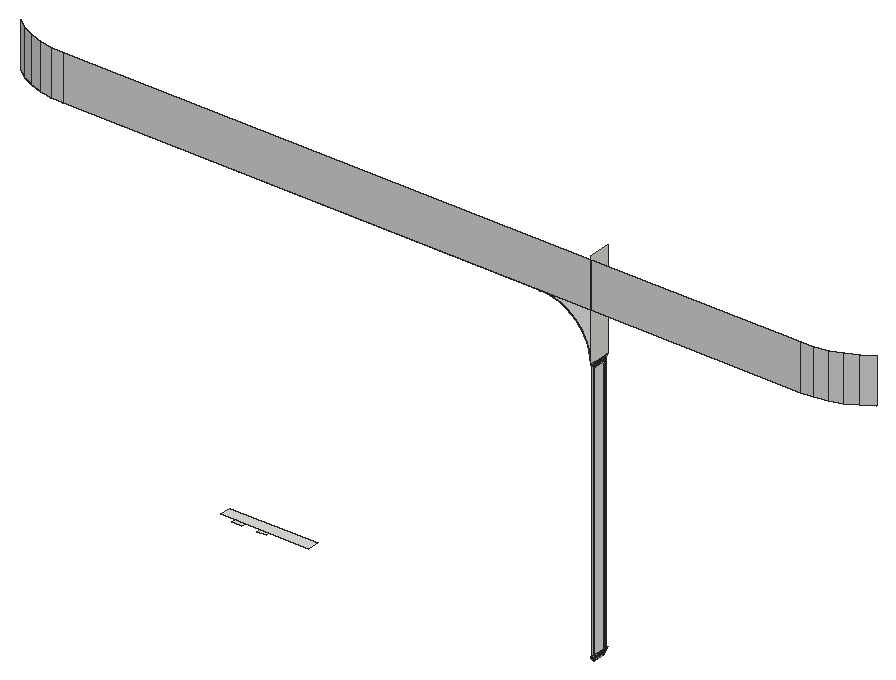
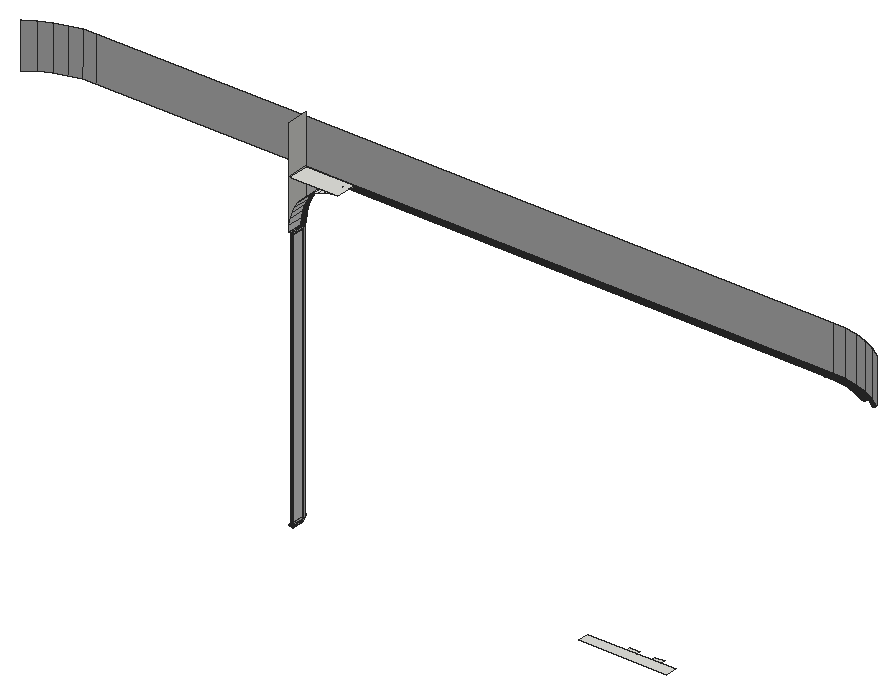
# SketchUp Ruby script. Lengths in inches.
U = 1.inch
M = Sketchup.active_model
def pt(a) = Geom::Point3d.new(a.map { |v| v * U })
def face(e, loops, mat)
  f = e.add_face(loops[0].map { |a| pt(a) })
  loops[1..].each { |l| e.add_face(l.map { |a| pt(a) }).erase! }
  f.material = f.back_material = mat if mat
  f
end
# faces: each face lists its corners as indices into pts; further lists are holes
def faces(e, pts, list, mat = nil) = list.each { |f| face(e, (f[0].is_a?(Array) ? f : [f]).map { |l| l.map { |i| pts[i] } }, mat) }
# xy, xz, yz: faces in a plane at the given z, y or x. An outline is a flat list of corners, or four numbers for a rectangle; further outlines are holes
def ring(l) = l.size == 4 ? [[l[0], l[1]], [l[2], l[1]], [l[2], l[3]], [l[0], l[3]]] : l.each_slice(2).to_a
def flat(e, list, mat, &to3) = list.each { |f| face(e, (f[0].is_a?(Array) ? f : [f]).map { |l| ring(l).map { |u, v| to3.(u, v) } }, mat) }
def xy(e, z, list, mat = nil) = flat(e, list, mat) { |x, y| [x, y, z] }
def xz(e, y, list, mat = nil) = flat(e, list, mat) { |x, z| [x, y, z] }
def yz(e, x, list, mat = nil) = flat(e, list, mat) { |y, z| [x, y, z] }
def lines(e, pts, list) = list.each { |a, b| e.add_line(pt(pts[a]), pt(pts[b])) }
# prism: a flat outline (further loops are holes) pulled along v
def prism(e, loops, v, mat = nil)
  f = face(e, loops, mat); d = Geom::Vector3d.new(v.map { |x| x * U })
  f.pushpull(f.normal.samedirection?(d) ? d.length : -d.length)
end
def box(e, o, s, mat = nil) = prism(e, [[o, [o[0] + s[0], o[1], o[2]], [o[0] + s[0], o[1] + s[1], o[2]], [o[0], o[1] + s[1], o[2]]]], [0, 0, s[2]], mat)
def at(x, y, z, deg = 0) = Geom::Transformation.translation(pt([x, y, z])) * Geom::Transformation.rotation(ORIGIN, Z_AXIS, deg.degrees)
def axes(o, x, y, z) = Geom::Transformation.new([*x, 0, *y, 0, *z, 0, *pt(o).to_a, 1])
def part(name) = M.definitions.add(name)
# library, detail: a bought-in or finely detailed component or shape, given as its bounding box
def library(name, o, s) = part(name).tap { |d| box(d.entities, o, s) }
def detail(e, o, s) = box(e.add_group.entities, o, s)
def put(e, d, t, mat = nil) = e.add_instance(d, t).tap { |i| i.material = mat if mat }
def group(e, t, mat = nil) = e.add_group.tap { |g| g.transformation = t; g.material = mat if mat }.entities
root = M.entities
M.materials.add("[Cladding Stucco White]").color = [200, 200, 200]
M.materials.add("[Color M01]").color = [226, 226, 226]
xy(root,162,[[65.53,1.33,67.97,2.33],[71.53,1.33,73.97,2.33],[61.97,2.33,83.6,5.0625]])
xy(root,239.79,[[24.28,1.78,21.22,1.98,21.24,2.14,24.28,1.9375],[24.28,1.78,24.28,1.9375,142,1.9375,142.01,1.78],[142.01,1.78,142,1.9375,142.02,1.9375,142.02,1.78],[24.28,1.9375,21.24,2.14,21.26,2.3,24.29,2.1],[24.28,1.9375,24.29,2.1,142.01,2.1,142,1.9375],
  [142,1.9375,142.01,2.1,142.02,2.1,142.02,1.9375],[21.22,1.98,18.24,2.57,18.28,2.73,21.24,2.14],[21.24,2.14,18.28,2.73,18.32,2.88,21.26,2.3],[18.24,2.57,15.36,3.55,15.43,3.69,18.28,2.73],[18.28,2.73,15.43,3.69,15.49,3.84,18.32,2.88],
  [15.36,3.55,12.64,4.89,12.72,5.03,15.43,3.69],[15.43,3.69,12.72,5.03,12.8,5.17,15.49,3.84]])
xy(root,240,[[142.02,1,154.02,6.39]])
xz(root,1,[[24.25,240,154.02,251.0625],[154.02,240,205.875,251.0625]],"[Cladding Stucco White]")
xz(root,1,[[154.02,228,154.02,240,142.02,240,143.58,239.9,145.125,239.59,146.61,239.09,148.02,238.39,149.32,237.52,150.5,236.49,151.54,235.31,152.41,234,153.11,232.59,153.61,231.11,153.92,229.57]],"[Color M01]")
yz(root,142.02,[[1.78,239.79,2.1,239.79,2.26,239.8125,2.42,239.84,2.57,239.88,2.73,239.9375,2.875,240,1,240,1.15,239.9375,1.3,239.88,1.46,239.84,1.62,239.8125]])
yz(root,153.96,[[1.78,162.55,1.67,162.67,5.73,162.67,5.61,162.55],[5.61,162.55,5.61,227.22,5.73,227.33,5.73,162.67],[1.67,162.67,1.55,162.78,5.84,162.78,5.73,162.67]])
yz(root,153.96,[[1.78,162.55,1.67,162.67,1.67,227.33,1.78,227.22]],"[Cladding Stucco White]")
yz(root,153.96,[[1.78,227.22,1.67,227.33,5.73,227.33,5.61,227.22],[1.67,227.33,1.55,227.45,5.84,227.45,5.73,227.33]],"[Color M01]")
yz(root,154.02,[[1,228,6.39,240],[1,240,6.39,252]])
yz(root,154.02,[[2.33,163.33,5.0625,226.67]],"[Color M01]")
p = [[154.02,2.33,163.33],[154.02,2.33,162],[154,2.22,162.11],[154,2.22,163.22],[154,2.22,226.78],[154.02,2.33,226.67],
  [154,5.17,162.11],[154.02,5.0625,162],[154,5.17,163.22],[154.02,5.0625,163.33],[154.02,5.0625,226.67],[154,5.17,226.78],
  [153.99,2.11,162.22],[153.99,2.11,163.11],[153.99,2.11,226.89],[153.99,5.28,162.22],[153.99,5.28,163.11],[153.99,5.28,226.89],
  [153.98,2,162.33],[153.98,2,163],[153.98,2,227],[153.98,5.39,162.33],[153.98,5.39,163],[153.98,5.39,227],
  [153.97,1.89,162.44],[153.97,1.89,162.89],[153.97,1.89,227.11],[153.97,5.5,162.44],[153.97,5.5,162.89],[153.97,5.5,227.11],
  [153.96,1.78,162.55],[153.96,1.78,162.78],[153.96,1.78,227.22],[153.96,5.61,162.55],[153.96,5.61,162.78],[153.96,5.61,227.22],
  [153.97,5.95,162.89],[153.96,5.84,162.78],[153.96,1.55,162.78],[153.97,1.44,162.89],[153.98,6.06,163],[153.98,1.33,163],
  [153.99,6.17,163.11],[153.99,1.22,163.11],[154,6.28,163.22],[154,1.11,163.22],[154.02,6.39,163.33],[154.02,1,163.33],
  [153.96,1.55,227.45],[153.97,1.44,227.56],[153.97,5.95,227.56],[153.96,5.84,227.45],[153.98,1.33,227.67],[153.98,6.06,227.67],
  [153.99,1.22,227.78],[153.99,6.17,227.78],[154,1.11,227.89],[154,6.28,227.89],[154.02,1,228],[154.02,2.875,228],
  [154.02,6.39,228],[153.95,1.15,228],[153.9,1.3,227.99],[153.86,1.46,227.99],[153.83,1.62,227.99],[153.8125,1.78,227.99],
  [153.81,1.9375,227.99],[153.8125,2.1,227.99],[153.83,2.26,227.99],[153.86,2.42,227.99],[153.9,2.57,227.99],[153.95,2.73,228],
  [153.92,1,229.57],[153.85,1.15,229.56],[153.8,1.3,229.55],[153.76,1.46,229.55],[153.73,1.62,229.54],[153.71,1.78,229.54],
  [153.71,1.9375,229.54],[153.71,2.1,229.54],[153.73,2.26,229.54],[153.76,2.42,229.55],[153.8,2.57,229.55],[153.85,2.73,229.56],
  [153.92,2.875,229.57],[153.92,6.39,229.57],[153.5,1.3,231.08],[153.46,1.46,231.06],[153.43,1.62,231.06],[153.41,1.78,231.05],
  [153.4,1.9375,231.05],[153.41,2.1,231.05],[153.43,2.26,231.06],[153.46,2.42,231.06],[153.5,2.57,231.08],[153.61,1,231.11],
  [153.55,1.15,231.09],[153.55,2.73,231.09],[153.61,2.875,231.11],[153.61,6.39,231.11],[153.11,1,232.59],[153.05,1.15,232.57],
  [153,1.3,232.55],[152.96,1.46,232.53],[152.93,1.62,232.52],[152.91,1.78,232.51],[152.91,1.9375,232.51],[152.91,2.1,232.51],
  [152.93,2.26,232.52],[152.96,2.42,232.53],[153,2.57,232.55],[153.05,2.73,232.57],[153.11,2.875,232.59],[153.11,6.39,232.59],
  [152.36,1.15,233.97],[152.31,1.3,233.94],[152.27,1.46,233.92],[152.25,1.62,233.91],[152.23,1.78,233.9],[152.23,1.9375,233.89],
  [152.23,2.1,233.9],[152.25,2.26,233.91],[152.27,2.42,233.92],[152.31,2.57,233.94],[152.36,2.73,233.97],[152.41,1,234],
  [152.41,2.875,234],[152.41,6.39,234],[151.49,1.15,235.27],[151.45,1.3,235.23],[151.41,1.46,235.21],[151.39,1.62,235.19],
  [151.375,1.78,235.18],[151.37,1.9375,235.18],[151.375,2.1,235.18],[151.39,2.26,235.19],[151.41,2.42,235.21],[151.45,2.57,235.23],
  [151.49,2.73,235.27],[151.54,1,235.31],[151.54,2.875,235.31],[151.54,6.39,235.31],[150.46,1.15,236.44],[150.42,1.3,236.4],
  [150.39,1.46,236.375],[150.37,1.62,236.35],[150.36,1.78,236.34],[150.35,1.9375,236.34],[150.36,2.1,236.34],[150.37,2.26,236.35],
  [150.39,2.42,236.375],[150.42,2.57,236.4],[150.46,2.73,236.44],[150.5,1,236.49],[150.5,2.875,236.49],[150.5,6.39,236.49],
  [149.21,1.62,237.37],[149.2,1.78,237.36],[149.19,1.9375,237.35],[149.2,2.1,237.36],[149.21,2.26,237.37],[149.32,1,237.52],
  [149.28,1.15,237.47],[149.25,1.3,237.43],[149.23,1.46,237.39],[149.23,2.42,237.39],[149.25,2.57,237.43],[149.28,2.73,237.47],
  [149.32,2.875,237.52],[149.32,6.39,237.52],[147.99,1.15,238.34],[147.96,1.3,238.29],[147.9375,1.46,238.26],[147.92,1.62,238.23],
  [147.92,1.78,238.21],[147.91,1.9375,238.21],[147.92,2.1,238.21],[147.92,2.26,238.23],[147.9375,2.42,238.26],[147.96,2.57,238.29],
  [147.99,2.73,238.34],[148.02,1,238.39],[148.02,2.875,238.39],[148.02,6.39,238.39],[146.55,1.46,238.94],[146.54,1.62,238.91],
  [146.53,1.78,238.9],[146.53,1.9375,238.89],[146.53,2.1,238.9],[146.54,2.26,238.91],[146.55,2.42,238.94],[146.61,1,239.09],
  [146.59,1.15,239.03],[146.57,1.3,238.98],[146.57,2.57,238.98],[146.59,2.73,239.03],[146.61,2.875,239.09],[146.61,6.39,239.09],
  [145.09,1.3,239.48],[145.08,1.46,239.4375],[145.08,1.62,239.41],[145.07,1.78,239.39],[145.07,1.9375,239.39],[145.07,2.1,239.39],
  [145.08,2.26,239.41],[145.08,2.42,239.4375],[145.09,2.57,239.48],[145.125,1,239.59],[145.11,1.15,239.53],[145.11,2.73,239.53],
  [145.125,2.875,239.59],[145.125,6.39,239.59],[143.57,1.3,239.78],[143.5625,1.46,239.74],[143.56,1.62,239.71],[143.56,1.78,239.69],
  [143.56,1.9375,239.6875],[143.56,2.1,239.69],[143.56,2.26,239.71],[143.5625,2.42,239.74],[143.57,2.57,239.78],[143.58,1,239.9],
  [143.58,1.15,239.83],[143.58,2.73,239.83],[143.58,2.875,239.9],[143.58,6.39,239.9],[142.02,1.3,239.88],[142.02,1.46,239.84],
  [142.02,1.62,239.8125],[142.02,1.78,239.79],[142.02,1.9375,239.79],[142.02,2.1,239.79],[142.02,2.26,239.8125],[142.02,2.42,239.84],
  [142.02,2.57,239.88],[142.02,1,240],[142.02,1.15,239.9375],[24.26,1.46,239.84],[24.26,1.3,239.88],[21.16,1.5,239.88],
  [21.18,1.66,239.84],[142.01,1.46,239.84],[142.01,1.3,239.88],[18.12,2.11,239.88],[18.16,2.26,239.84],[24.27,1.62,239.8125],
  [21.2,1.82,239.8125],[142.01,1.62,239.8125],[24.28,1.78,239.79],[21.22,1.98,239.79],[142.01,1.78,239.79],[18.2,2.41,239.8125],
  [18.24,2.57,239.79],[15.18,3.11,239.88],[15.24,3.25,239.84],[24.29,2.26,239.8125],[24.29,2.1,239.79],[21.26,2.3,239.79],
  [21.28,2.46,239.8125],[142.01,2.26,239.8125],[142.01,2.1,239.79],[15.3,3.4,239.8125],[18.32,2.88,239.79],[18.36,3.04,239.8125],
  [24.3,2.42,239.84],[21.3,2.61,239.84],[142.01,2.42,239.84],[15.36,3.55,239.79],[24.3,2.57,239.88],[21.32,2.77,239.88],
  [142.01,2.57,239.88],[18.41,3.19,239.84],[18.45,3.34,239.88],[142.02,2.73,239.9375],[142.02,2.875,240],[15.49,3.84,239.79],
  [15.55,3.99,239.8125],[15.61,4.14,239.84],[12.4,4.48,239.88],[12.48,4.61,239.84],[12.56,4.75,239.8125],[15.67,4.28,239.88],
  [12.64,4.89,239.79],[12.8,5.17,239.79],[12.88,5.31,239.8125],[12.96,5.45,239.84],[13.04,5.58,239.88],[9.82,6.2,239.88],
  [9.92,6.32,239.84],[10.02,6.45,239.8125],[24.25,1.15,239.9375],[24.25,1,240],[21.12,1.21,240],[21.14,1.35,239.9375],
  [142.01,1.15,239.9375],[18.04,1.82,240],[18.08,1.96,239.9375],[15.07,2.83,240],[15.12,2.96,239.9375],[24.31,2.73,239.9375],
  [21.34,2.92,239.9375],[142.01,2.73,239.9375],[24.3125,2.875,240],[21.36,3.07,240],[12.25,4.22,240],[12.32,4.34,239.9375],
  [18.49,3.49,239.9375],[18.52,3.63,240],[142.02,6.39,240],[15.73,4.43,239.9375],[15.78,4.5625,240],[9.64,5.96,240],
  [9.73,6.08,239.9375],[13.12,5.71,239.9375],[13.19,5.84,240],[21.12,1.21,251.0625],[24.25,1,251.0625],[205.875,1,251.0625],
  [205.875,1,240],[209.01,1.21,240],[209.01,1.21,251.0625],[208.3,1.16,251.0625],[18.04,1.82,251.0625],[212.09,1.82,240],
  [212.09,1.82,251.0625],[15.07,2.83,251.0625],[215.06,2.83,240],[215.06,2.83,251.0625],[12.25,4.22,251.0625],[217.875,4.22,240],
  [217.875,4.22,251.0625],[9.64,5.96,251.0625],[220.49,5.96,240],[220.49,5.96,251.0625]]
faces(root,p,[[0,1,2,3,4,5],[3,2,12,13,14,4],[13,12,18,19,20,14],[19,18,24,25,26,20],[25,24,30,31,32,26],[315,292,291,316],[317,318,319,320,321],[322,295,292,315],
  [320,319,323,324],[325,297,295,322],[324,323,326,327],[328,304,297,325],[327,326,329,330],[331,311,304,328],[330,329,332,333]],"[Cladding Stucco White]")
faces(root,p,[[6,7,1,2],[8,6,7,9,10,11],[15,6,2,12],[16,15,6,8,11,17],[21,15,12,18],[22,21,15,16,17,23],[27,21,18,24],[28,27,21,22,23,29],
  [33,27,24,30],[34,33,27,28,29,35],[36,37,34,31,38,39,25,28],[40,36,28,25,39,41,19,22],[42,40,22,19,41,43,13,16],[44,42,16,13,43,45,3,8],[46,44,8,3,45,47,0,9],[61,62,63,64,65,66,67,68,69,70,71,59,58],
  [237,238,239,240],[237,241,242,238],[226,242,241,227],[240,239,243,244],[245,237,240,246],[245,247,241,237],[227,241,247,228],[248,245,246,249],
  [248,250,247,245],[228,247,250,229],[246,240,244,251],[249,246,251,252],[244,243,253,254],[255,256,257,258],[255,259,260,256],[231,260,259,232],
  [251,244,254,261],[258,257,262,263],[264,255,258,265],[264,266,259,255],[232,259,266,233],[252,251,261,267],[268,264,265,269],[268,270,266,264],
  [233,266,270,234],[265,258,263,271],[269,265,271,272],[263,262,275,276],[271,263,276,277],[254,253,278,279],[261,254,279,280],[272,271,277,281],
  [267,261,280,282],[276,275,283,284],[277,276,284,285],[281,277,285,286],[279,278,287,288],[280,279,288,289],[290,291,292,293],[290,294,235,291],
  [236,235,294],[238,290,293,239],[238,242,294,290],[236,294,242,226],[293,292,295,296],[239,293,296,243],[296,295,297,298],[243,296,298,253],
  [299,268,269,300],[299,301,270,268],[234,270,301,273],[302,299,300,303],[302,274,301,299],[273,301,274],[298,297,304,305],[300,269,272,306],
  [303,300,306,307],[253,298,305,278],[306,272,281,309],[307,306,309,310],[305,304,311,312],[278,305,312,287],[309,281,286,313],[310,309,313,314]])
faces(root,p,[[5,4,11,10],[4,14,17,11],[14,20,23,17],[20,26,29,23],[26,32,35,29],[48,49,50,51],[49,52,53,50],[52,54,55,53],
  [54,56,57,55],[56,58,59,60,57],[61,58,72,73],[62,61,73,74],[63,62,74,75],[64,63,75,76],[65,64,76,77],[66,65,77,78],
  [67,66,78,79],[68,67,79,80],[69,68,80,81],[70,69,81,82],[71,70,82,83],[59,71,83,84],[84,85,60,59],[75,74,86,87],
  [76,75,87,88],[77,76,88,89],[78,77,89,90],[79,78,90,91],[80,79,91,92],[81,80,92,93],[82,81,93,94],[73,72,95,96],
  [74,73,96,86],[83,82,94,97],[84,83,97,98],[98,99,85,84],[96,95,100,101],[86,96,101,102],[87,86,102,103],[88,87,103,104],
  [89,88,104,105],[90,89,105,106],[91,90,106,107],[92,91,107,108],[93,92,108,109],[94,93,109,110],[97,94,110,111],[98,97,111,112],
  [112,113,99,98],[102,101,114,115],[103,102,115,116],[104,103,116,117],[105,104,117,118],[106,105,118,119],[107,106,119,120],[108,107,120,121],
  [109,108,121,122],[110,109,122,123],[111,110,123,124],[101,100,125,114],[112,111,124,126],[126,127,113,112],[115,114,128,129],[116,115,129,130],
  [117,116,130,131],[118,117,131,132],[119,118,132,133],[120,119,133,134],[121,120,134,135],[122,121,135,136],[123,122,136,137],[124,123,137,138],
  [114,125,139,128],[126,124,138,140],[140,141,127,126],[129,128,142,143],[130,129,143,144],[131,130,144,145],[132,131,145,146],[133,132,146,147],
  [134,133,147,148],[135,134,148,149],[136,135,149,150],[137,136,150,151],[138,137,151,152],[128,139,153,142],[140,138,152,154],[154,155,141,140],
  [146,145,156,157],[147,146,157,158],[148,147,158,159],[149,148,159,160],[142,153,161,162],[143,142,162,163],[144,143,163,164],[145,144,164,156],
  [150,149,160,165],[151,150,165,166],[152,151,166,167],[154,152,167,168],[168,169,155,154],[163,162,170,171],[164,163,171,172],[156,164,172,173],
  [157,156,173,174],[158,157,174,175],[159,158,175,176],[160,159,176,177],[165,160,177,178],[166,165,178,179],[167,166,179,180],[162,161,181,170],
  [168,167,180,182],[182,183,169,168],[173,172,184,185],[174,173,185,186],[175,174,186,187],[176,175,187,188],[177,176,188,189],[178,177,189,190],
  [170,181,191,192],[171,170,192,193],[172,171,193,184],[179,178,190,194],[180,179,194,195],[182,180,195,196],[196,197,183,182],[184,193,198,199],
  [185,184,199,200],[186,185,200,201],[187,186,201,202],[188,187,202,203],[189,188,203,204],[190,189,204,205],[194,190,205,206],[192,191,207,208],
  [193,192,208,198],[195,194,206,209],[196,195,209,210],[210,211,197,196],[199,198,212,213],[200,199,213,214],[201,200,214,215],[202,201,215,216],
  [203,202,216,217],[204,203,217,218],[205,204,218,219],[206,205,219,220],[208,207,221,222],[198,208,222,212],[209,206,220,223],[210,209,223,224],
  [224,225,211,210],[212,226,227,213],[213,227,228,214],[214,228,229,215],[215,229,230,216],[216,230,231,217],[217,231,232,218],[218,232,233,219],
  [219,233,234,220],[221,235,236,222],[222,236,226,212],[220,234,273,223],[223,273,274,224],[274,308,225,224]],"[Color M01]")
